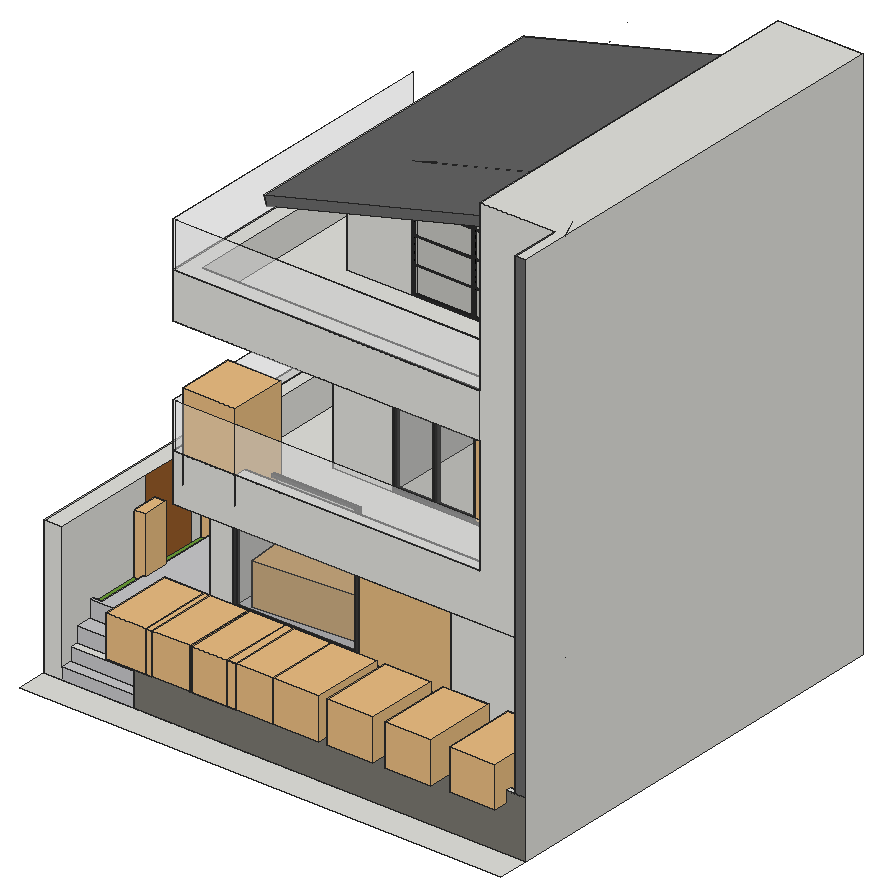
# SketchUp Ruby script. Lengths in inches.
U = 1.inch
M = Sketchup.active_model
def pt(a) = Geom::Point3d.new(a.map { |v| v * U })
def face(e, loops, mat)
  f = e.add_face(loops[0].map { |a| pt(a) })
  loops[1..].each { |l| e.add_face(l.map { |a| pt(a) }).erase! }
  f.material = f.back_material = mat if mat
  f
end
# faces: each face lists its corners as indices into pts; further lists are holes
def faces(e, pts, list, mat = nil) = list.each { |f| face(e, (f[0].is_a?(Array) ? f : [f]).map { |l| l.map { |i| pts[i] } }, mat) }
# xy, xz, yz: faces in a plane at the given z, y or x. An outline is a flat list of corners, or four numbers for a rectangle; further outlines are holes
def ring(l) = l.size == 4 ? [[l[0], l[1]], [l[2], l[1]], [l[2], l[3]], [l[0], l[3]]] : l.each_slice(2).to_a
def flat(e, list, mat, &to3) = list.each { |f| face(e, (f[0].is_a?(Array) ? f : [f]).map { |l| ring(l).map { |u, v| to3.(u, v) } }, mat) }
def xy(e, z, list, mat = nil) = flat(e, list, mat) { |x, y| [x, y, z] }
def xz(e, y, list, mat = nil) = flat(e, list, mat) { |x, z| [x, y, z] }
def yz(e, x, list, mat = nil) = flat(e, list, mat) { |y, z| [x, y, z] }
def lines(e, pts, list) = list.each { |a, b| e.add_line(pt(pts[a]), pt(pts[b])) }
# prism: a flat outline (further loops are holes) pulled along v
def prism(e, loops, v, mat = nil)
  f = face(e, loops, mat); d = Geom::Vector3d.new(v.map { |x| x * U })
  f.pushpull(f.normal.samedirection?(d) ? d.length : -d.length)
end
def box(e, o, s, mat = nil) = prism(e, [[o, [o[0] + s[0], o[1], o[2]], [o[0] + s[0], o[1] + s[1], o[2]], [o[0], o[1] + s[1], o[2]]]], [0, 0, s[2]], mat)
def at(x, y, z, deg = 0) = Geom::Transformation.translation(pt([x, y, z])) * Geom::Transformation.rotation(ORIGIN, Z_AXIS, deg.degrees)
def axes(o, x, y, z) = Geom::Transformation.new([*x, 0, *y, 0, *z, 0, *pt(o).to_a, 1])
def part(name) = M.definitions.add(name)
# library, detail: a bought-in or finely detailed component or shape, given as its bounding box
def library(name, o, s) = part(name).tap { |d| box(d.entities, o, s) }
def detail(e, o, s) = box(e.add_group.entities, o, s)
def put(e, d, t, mat = nil) = e.add_instance(d, t).tap { |i| i.material = mat if mat }
def group(e, t, mat = nil) = e.add_group.tap { |g| g.transformation = t; g.material = mat if mat }.entities
root = M.entities
M.materials.add("Glass_Window_Neutral\#2").color = [0, 0, 0]
M.materials["Glass_Window_Neutral\#2"].alpha = 0.125
M.materials.add("Iron_Blurry_5cm").color = [3, 3, 3]
M.materials.add("Resin FOG").color = [255, 255, 255]
M.materials["Resin FOG"].alpha = 0.29
M.materials.add("[0134_DimGray]").color = [105, 105, 105]
M.materials.add("[Color M07]").color = [58, 58, 58]
M.materials.add("[Color M09]4").color = [0, 0, 0]
M.materials.add("[Grass Dark Green]").color = [106, 157, 55]
M.materials.add("[Polished Concrete New]").color = [200, 200, 203]
M.materials.add("[Rough Square Concrete Block]").color = [123, 120, 113]
M.materials.add("[Slate]").color = [102, 110, 108]
M.materials.add("[Translucent Glass Gray]3").color = [128, 128, 128]
M.materials["[Translucent Glass Gray]3"].alpha = 0.3
M.materials.add("[Wood Floor Dark]").color = [153, 94, 42]
c1 = library("Door+Glass",[-5.91,-81.85,0],[24.58,33.9,83.07])
c2 = part("WINDOW (3)")
xy(c2.entities,0,[[0,0,59.06,1.97]],"[Color M07]")
xy(c2.entities,1.97,[[1.97,0,57.09,0.98],[1.97,0.98,57.09,1.97]],"[Color M07]")
xy(c2.entities,104.33,[[1.97,0,57.09,0.98],[1.97,0.98,57.09,1.97]],"[Color M07]")
xy(c2.entities,106.3,[[0,0,59.06,1.97]],"[Color M07]")
xz(c2.entities,0,[[[0,0,59.06,106.3],[1.97,1.97,57.09,104.33]]],"[Color M07]")
xz(c2.entities,0.98,[[1.97,1.97,57.09,104.33]],"[Translucent Glass Gray]3")
xz(c2.entities,1.97,[[[0,0,59.06,106.3],[1.97,1.97,57.09,104.33]]],"[Color M07]")
yz(c2.entities,0,[[0,0,1.97,106.3]],"[Color M07]")
yz(c2.entities,1.97,[[0,1.97,0.98,104.33],[0.98,1.97,1.97,104.33]],"[Color M07]")
yz(c2.entities,57.09,[[0,1.97,0.98,104.33],[0.98,1.97,1.97,104.33]],"[Color M07]")
yz(c2.entities,59.06,[[0,0,1.97,106.3]],"[Color M07]")
c3 = part("glass")
p = [[-167.89,-148.66,14.5],[-167.89,-148.66,14.51],[-167.89,-148.66,14.52]]
lines(c3.entities,p,[[0,1],[1,2]])
g1 = group(c3.entities,at(-34.63,-28.25,2))
box(g1,[0,0,0],[93.3125,0.375,32.75],"Resin FOG")
c4 = part("Component\#72")
g2 = group(c4.entities,at(0,26.17,94.49),"[Color M09]4")
xy(g2,-94.49,[[0,-26.17,1.18,0]],"Iron_Blurry_5cm")
xy(g2,-93.8,[[0,-25.51,0.59,-0.67],[0.59,-25.51,1.18,-0.67]],"Iron_Blurry_5cm")
xy(g2,-70.52,[[0.59,-25.51,1.18,-0.67]],"Iron_Blurry_5cm")
xy(g2,-69.84,[[0.59,-25.51,1.18,-0.67]],"Iron_Blurry_5cm")
xy(g2,-47.24,[[0.59,-25.51,1.18,-0.67]],"Iron_Blurry_5cm")
xy(g2,-46.56,[[0.59,-25.51,1.18,-0.67]],"Iron_Blurry_5cm")
xy(g2,-23.97,[[0.59,-25.51,1.18,-0.67]],"Iron_Blurry_5cm")
xy(g2,-23.28,[[0.59,-25.51,1.18,-0.67]],"Iron_Blurry_5cm")
xy(g2,-0.6875,[[0,-25.51,0.59,-0.67],[0.59,-25.51,1.18,-0.67]],"Iron_Blurry_5cm")
xy(g2,0,[[0,-26.17,1.18,0]],"Iron_Blurry_5cm")
xz(g2,-26.17,[[0,-94.49,1.18,0]],"Iron_Blurry_5cm")
xz(g2,-25.51,[[0,-93.8,0.59,-0.6875],[0.59,-93.8,1.18,-70.52],[0.59,-70.52,1.18,-69.84],[0.59,-69.84,1.18,-47.24],[0.59,-47.24,1.18,-46.56],
  [0.59,-46.56,1.18,-23.97],[0.59,-23.97,1.18,-23.28],[0.59,-23.28,1.18,-0.6875]],"Iron_Blurry_5cm")
xz(g2,-0.67,[[0,-93.8,0.59,-0.6875],[0.59,-93.8,1.18,-70.52],[0.59,-70.52,1.18,-69.84],[0.59,-69.84,1.18,-47.24],[0.59,-47.24,1.18,-46.56],
  [0.59,-46.56,1.18,-23.97],[0.59,-23.97,1.18,-23.28],[0.59,-23.28,1.18,-0.6875]],"Iron_Blurry_5cm")
xz(g2,0,[[0,-94.49,1.18,0]],"Iron_Blurry_5cm")
yz(g2,0,[[[-26.17,-94.49,0,0],[-25.51,-93.8,-0.67,-0.6875]]],"Iron_Blurry_5cm")
yz(g2,0.59,[[-25.51,-93.8,-0.67,-70.52],[-25.51,-69.84,-0.67,-47.24],[-25.51,-46.56,-0.67,-23.97],[-25.51,-23.28,-0.67,-0.6875]],"Glass_Window_Neutral\#2")
yz(g2,0.59,[[-25.51,-70.52,-0.67,-69.84],[-25.51,-47.24,-0.67,-46.56],[-25.51,-23.97,-0.67,-23.28]],"Iron_Blurry_5cm")
yz(g2,1.18,[[[-26.17,-94.49,0,0],[-25.51,-93.8,-0.67,-0.6875]],[-25.51,-70.52,-0.67,-69.84],[-25.51,-47.24,-0.67,-46.56],[-25.51,-23.97,-0.67,-23.28]],"Iron_Blurry_5cm")
g3 = group(c4.entities,at(0,52.35,94.49),"[Color M09]4")
xy(g3,-94.49,[[0,-26.17,1.18,0]],"Iron_Blurry_5cm")
xy(g3,-93.8,[[0,-25.51,0.59,-0.67],[0.59,-25.51,1.18,-0.67]],"Iron_Blurry_5cm")
xy(g3,-70.52,[[0.59,-25.51,1.18,-0.67]],"Iron_Blurry_5cm")
xy(g3,-69.84,[[0.59,-25.51,1.18,-0.67]],"Iron_Blurry_5cm")
xy(g3,-47.24,[[0.59,-25.51,1.18,-0.67]],"Iron_Blurry_5cm")
xy(g3,-46.56,[[0.59,-25.51,1.18,-0.67]],"Iron_Blurry_5cm")
xy(g3,-23.97,[[0.59,-25.51,1.18,-0.67]],"Iron_Blurry_5cm")
xy(g3,-23.28,[[0.59,-25.51,1.18,-0.67]],"Iron_Blurry_5cm")
xy(g3,-0.6875,[[0,-25.51,0.59,-0.67],[0.59,-25.51,1.18,-0.67]],"Iron_Blurry_5cm")
xy(g3,0,[[0,-26.17,1.18,0]],"Iron_Blurry_5cm")
xz(g3,-26.17,[[0,-94.49,1.18,0]],"Iron_Blurry_5cm")
xz(g3,-25.51,[[0,-93.8,0.59,-0.6875],[0.59,-93.8,1.18,-70.52],[0.59,-70.52,1.18,-69.84],[0.59,-69.84,1.18,-47.24],[0.59,-47.24,1.18,-46.56],
  [0.59,-46.56,1.18,-23.97],[0.59,-23.97,1.18,-23.28],[0.59,-23.28,1.18,-0.6875]],"Iron_Blurry_5cm")
xz(g3,-0.67,[[0,-93.8,0.59,-0.6875],[0.59,-93.8,1.18,-70.52],[0.59,-70.52,1.18,-69.84],[0.59,-69.84,1.18,-47.24],[0.59,-47.24,1.18,-46.56],
  [0.59,-46.56,1.18,-23.97],[0.59,-23.97,1.18,-23.28],[0.59,-23.28,1.18,-0.6875]],"Iron_Blurry_5cm")
xz(g3,0,[[0,-94.49,1.18,0]],"Iron_Blurry_5cm")
yz(g3,0,[[[-26.17,-94.49,0,0],[-25.51,-93.8,-0.67,-0.6875]]],"Iron_Blurry_5cm")
yz(g3,0.59,[[-25.51,-93.8,-0.67,-70.52],[-25.51,-69.84,-0.67,-47.24],[-25.51,-46.56,-0.67,-23.97],[-25.51,-23.28,-0.67,-0.6875]],"Glass_Window_Neutral\#2")
yz(g3,0.59,[[-25.51,-70.52,-0.67,-69.84],[-25.51,-47.24,-0.67,-46.56],[-25.51,-23.97,-0.67,-23.28]],"Iron_Blurry_5cm")
yz(g3,1.18,[[[-26.17,-94.49,0,0],[-25.51,-93.8,-0.67,-0.6875]],[-25.51,-70.52,-0.67,-69.84],[-25.51,-47.24,-0.67,-46.56],[-25.51,-23.97,-0.67,-23.28]],"Iron_Blurry_5cm")
c5 = library("SOFA\#1",[0.35,-39.08,0.31],[80.46,34.29,30.24])
c6 = library("CURTAIN",[20.4,9.88,0],[29.77,2.88,102.36])
c7 = library("S21",[-74.41,-56.05,0],[89.11,79.55,33.18])
c8 = library("Broadleaf plant",[0,0,0],[149.19,166.1,98.1875])
c9 = library("cay+chuoi",[26.89,19.66,0.52],[41.96,45.65,69.71])
c10 = library("Group_2",[-1.28,-0.39,0],[21.22,20.51,48.44])
xy(root,0,[[0,0,384.5625,24.3],[0,24.3,370.25,361.1875],[370.25,24.3,384.5625,49.12],[370.25,49.12,384.5625,361.1875]])
xy(root,9.26,[[13.89,24.3,71.28,33.18]],"[Polished Concrete New]")
xy(root,15.375,[[75.74,28.76,380.11,44.66]])
xy(root,19.65,[[13.89,33.18,71.28,39.8]])
xy(root,31.63,[[13.89,39.8,71.28,52.87]],"[Polished Concrete New]")
xy(root,41.75,[[13.89,54.78,21.5625,334.58]],"[Grass Dark Green]")
xy(root,45.625,[[71.28,24.3,376.39,24.3,376.39,28.76,75.74,28.76,75.74,44.66,376.39,44.66,376.39,49.12,71.28,49.12],[376.39,24.3,380.11,28.76]])
xy(root,45.625,[[71.28,49.12,376.39,49.12,376.39,81.5,278.92,81.5,278.92,167.87,89.95,167.87,89.95,100.12,71.28,100.12,71.28,334.58,21.5625,334.58,21.5625,54.78,13.89,54.78,13.89,52.87,71.28,52.87]],"[Polished Concrete New]")
xy(root,45.625,[[376.39,28.76,380.11,44.66]],"[Slate]")
xy(root,109.1875,[[0,24.3,13.89,361.1875],[13.89,334.58,71.28,361.1875]])
xy(root,128.75,[[71.28,63.93,89.95,100.12],[89.95,63.93,168.05,167.87],[168.05,63.93,168.05,167.87,278.92,167.87,278.92,81.5,238.99,81.5,238.99,63.93],[238.99,63.93,318.92,81.5],[318.92,63.93,376.39,81.5]])
xy(root,138.125,[[81.53,73.41,316.72,73.41,316.72,148.24,277.01,148.24,277.01,335.05,179.52,335.05,179.52,148.24,131.1,148.24,131.1,340.9,81.53,340.9]])
xy(root,166.625,[[71.28,63.93,316.72,63.93,316.72,73.41,81.53,73.41,81.53,361.1875,71.28,361.1875]])
xy(root,259.91,[[179.52,148.24,277.01,335.05]])
xy(root,259.91,[[71.28,63.93,71.28,361.1875,81.53,361.1875,81.53,340.9,131.1,340.9,131.1,63.93],[131.1,63.93,316.72,148.24]],"[Wood Floor Dark]")
xy(root,270.4375,[[83.91,77.46,316.72,77.46,316.72,167.52,277.01,167.52,277.01,171.89,179.52,171.89,179.52,167.52,127.35,167.52,127.35,349.08,316.72,361.1875,83.91,361.1875],[127.35,349.08,316.72,349.08,316.72,361.1875]])
xy(root,295.9375,[[71.28,63.93,316.72,63.93,316.72,77.46,83.91,77.46,83.91,361.1875,71.28,361.1875]])
xy(root,430.4375,[[376.39,24.3,384.5625,24.3,384.5625,361.1875,316.72,361.1875,316.72,63.93,376.39,63.93]])
xz(root,24.3,[[0,0,13.89,109.1875]])
xz(root,24.3,[[376.39,45.625,384.5625,430.4375]],"[0134_DimGray]")
xz(root,24.3,[[13.89,0,71.28,9.26]],"[Polished Concrete New]")
xz(root,24.3,[[71.28,0,384.5625,45.625]],"[Rough Square Concrete Block]")
xz(root,28.76,[[75.74,15.375,380.11,45.625]])
xz(root,33.18,[[13.89,9.26,71.28,19.65]],"[Polished Concrete New]")
xz(root,39.8,[[13.89,19.65,71.28,31.63]],"[Polished Concrete New]")
xz(root,44.66,[[75.74,15.375,380.11,45.625]])
xz(root,52.87,[[13.89,31.63,71.28,45.625]],"[Polished Concrete New]")
xz(root,54.78,[[13.89,41.75,21.5625,45.625]],"[Polished Concrete New]")
xz(root,63.93,[[71.28,128.75,376.39,128.75,376.39,430.4375,316.72,430.4375,316.72,166.625,71.28,166.625],[71.28,259.91,316.72,295.9375]])
xz(root,73.41,[[81.53,138.125,316.72,166.625]])
xz(root,77.46,[[83.91,270.4375,316.72,295.9375]])
xz(root,81.5,[[278.92,45.625,376.39,128.75]])
xz(root,99.1,[[117.72,342.48,317.8,396.09,315.85,403.37,115.77,349.76]],"[0134_DimGray]")
xz(root,100.12,[[71.28,45.625,89.95,128.75]])
xz(root,148.24,[[131.1,138.125,179.52,259.91],[277.01,138.125,316.72,259.91]])
xz(root,167.52,[[127.35,270.4375,179.52,270.4375,179.52,359.04,277.01,385.16,277.01,270.4375,316.72,270.4375,316.72,395.1875,285.33,395.1875,239.34,382.88,191.55,370.0625,187.79,369.05,176.96,364.52,176.85,364.83,127.23,346.03,127.35,345.72],[187.79,369.05,191.55,370.0625,191.55,370.09,187.96,369.125],[191.55,370.0625,239.34,382.88,191.55,370.09],[191.55,370.0625,239.34,382.88,191.55,370.09]])
xz(root,167.87,[[89.95,45.625,164.47,128.75]])
xz(root,167.87,[[164.47,45.625,278.92,128.75]],"[Wood Floor Dark]")
xz(root,171.89,[[179.52,270.4375,277.01,270.4375,277.01,385.16,179.52,359.04]])
xz(root,334.58,[[13.89,41.75,21.5625,41.75,21.5625,45.625,71.28,45.625,71.28,109.1875,13.89,109.1875]])
xz(root,335.05,[[179.52,138.125,277.01,259.91]])
xz(root,340.9,[[81.53,138.125,131.1,259.91]])
xz(root,349.08,[[127.35,345.72,127.23,346.03,127.35,346.07],[127.35,345.72,127.35,346.07,176.85,364.83]])
xz(root,358.27,[[117.72,342.48,115.77,349.76,315.85,403.37,317.8,396.09]])
xz(root,361.1875,[[0,0,0,109.1875,71.28,109.1875,71.28,166.625,81.53,166.625,81.53,259.91,71.28,259.91,71.28,295.9375,83.91,295.9375,83.91,270.4375,142.5625,270.4375,142.5625,0],[142.5625,0,142.5625,270.4375,316.72,270.4375,316.72,430.4375,384.5625,430.4375,384.5625,0]])
yz(root,0,[[24.3,0,361.1875,109.1875]])
yz(root,13.89,[[24.3,9.26,33.18,9.26,33.18,19.65,39.8,19.65,39.8,31.63,52.87,31.63,52.87,45.625,54.78,45.625,54.78,41.75,107.85,41.75,107.85,109.1875,24.3,109.1875],[154.01,41.75,198.21,109.1875],[258.15,41.75,334.58,109.1875]])
yz(root,13.89,[[107.85,41.75,154.01,109.1875],[198.21,41.75,258.15,109.1875]],"[Wood Floor Dark]")
yz(root,21.5625,[[54.78,41.75,334.58,45.625]],"[Polished Concrete New]")
yz(root,71.28,[[24.3,0,24.3,9.26,33.18,9.26,33.18,12.26,49.12,12.26,49.12,0],[24.3,9.26,33.18,12.26],[24.3,12.26,33.18,21.58],[33.18,19.65,33.18,21.58,24.3,21.58,24.3,45.625,49.12,45.625,49.12,31.63,39.8,31.63,39.8,19.65],[39.8,24.52,49.12,31.63],
  [49.12,31.63,52.87,45.625],[100.12,45.625,100.12,128.75,63.93,128.75,63.93,166.625,361.1875,166.625,361.1875,109.1875,334.58,109.1875,334.58,45.625],[63.93,259.91,361.1875,295.9375]])
yz(root,75.74,[[28.76,15.375,44.66,45.625]])
yz(root,81.53,[[73.41,138.125,340.9,166.625],[340.9,166.625,361.1875,259.91]])
yz(root,83.91,[[77.46,270.4375,361.1875,295.9375]])
yz(root,89.95,[[100.12,45.625,167.87,128.75]])
yz(root,127.35,[[167.52,270.4375,349.08,345.72]])
yz(root,131.1,[[148.24,138.125,340.9,259.91]])
yz(root,179.52,[[148.24,138.125,335.05,259.91],[167.52,270.4375,171.89,358.25],[167.52,358.25,171.89,358.87],[167.52,358.87,171.89,359.04]])
yz(root,277.01,[[148.24,138.125,335.05,259.91],[167.52,270.4375,171.89,385.16]])
yz(root,278.92,[[81.5,45.625,167.87,128.75]])
yz(root,316.72,[[73.41,138.125,73.41,166.625,63.93,166.625,63.93,259.91,148.24,259.91,148.24,138.125],[77.46,270.4375,77.46,295.9375,63.93,295.9375,63.93,430.4375,361.1875,430.4375,361.1875,270.4375,349.08,270.4375,349.08,395.1875,167.52,395.1875,167.52,270.4375]])
yz(root,376.39,[[24.3,45.625,24.3,430.4375,63.93,430.4375,63.93,128.75,81.5,128.75,81.5,45.625]],"[0134_DimGray]")
yz(root,380.11,[[28.76,15.375,44.66,45.625]])
yz(root,384.5625,[[24.3,0,361.1875,430.4375]])
p = [[127.35,349.08,270.4375],[127.35,349.08,345.72],[127.35,349.08,346.07],[127.35,349.08,349.9],[316.72,361.1875,349.9],[316.72,361.1875,270.4375],
  [117.72,358.27,342.48],[117.72,99.1,342.48],[115.77,99.1,349.76],[115.77,358.27,349.76],[317.8,358.27,396.09],[317.8,99.1,396.09],
  [179.52,167.52,359.04],[277.01,167.52,385.16],[277.01,171.89,385.16],[179.52,171.89,359.04],[127.35,167.52,345.72],[127.23,167.52,346.03],
  [127.23,349.08,346.03],[176.85,167.52,364.83],[176.85,349.08,364.83],[315.85,99.1,403.37],[315.85,358.27,403.37],[176.96,167.52,364.52],
  [176.96,349.08,364.52],[316.72,349.08,395.1875],[285.33,349.08,395.1875],[191.55,167.52,369.1875],[191.55,167.52,370.0625],[191.55,349.95,376.35],
  [191.55,349.08,376.35],[178.89,167.52,358.87],[179.52,167.52,366.84],[187.79,167.52,369.05],[384.5625,63.93,430.4375],[376.39,81.5,430.4375],
  [376.39,81.5,128.75],[384.5625,63.93,128.75]]
faces(root,p,[[0,1,2,3,4,5],[6,7,8,9],[1,16,17,18],[18,17,19,20,2],[13,12,15,14],[23,24,20,19],[11,10,22,21]])
faces(root,p,[[[7,6,10,11],[12,13,14,15]]],"[Wood Floor Dark]")
faces(root,p,[[9,8,21,22]],"[0134_DimGray]")
lines(root,p,[[25,26],[27,28],[29,30],[12,31],[32,33],[34,35],[35,36],[36,37]])
put(root,c1,axes([53.29,120.77,45.625],[0.10626,0.99434,0],[-2.88358,0.30817,0],[0,0,1]))
put(root,c2,axes([89.95,100.12,45.625],[1.71,0,0],[0,1,0],[0,0,1]))
put(root,c3,axes([163.55,88.23,293.71],[2.60999,0,0],[0,0.86,0],[0,0,1.115]))
put(root,c3,axes([163.55,88.23,164.4],[2.60999,0,0],[0,0.86,0],[0,0,1.115]))
put(root,c3,axes([95.58,215.03,293.71],[0,-2.57471,0],[0.86,0,0],[0,0,1.115]))
put(root,c3,axes([95.58,215.03,164.4],[0,-2.57471,0],[0.86,0,0],[0,0,1.115]))
put(root,c4,axes([277.01,167.52,270.4375],[0,1,0],[-1.8623,0,0],[0,0,0.9044]))
put(root,c5,at(190.06,295.82,142.24))
put(root,c6,axes([222.82,104.33,140.38],[1.05822,0,0],[0,4.44245,0],[0,0,1.16768]))
put(root,c6,axes([227.52,145.53,261.63],[1,0,0],[0,2.22481,0],[0,0,0.92086]))
put(root,c7,axes([119.9375,145.91,45.625],[-0.03923,0.49846,0],[-0.99692,-0.07846,0],[0,0,1]))
put(root,c8,axes([65.69,4.17,42.14],[0.245,0,0],[0,0.35,0],[0,0,0.3332]))
put(root,c8,axes([97.5,4.17,42.14],[0.245,0,0],[0,0.35,0],[0,0,0.3332]))
put(root,c8,axes([132.81,4.17,42.14],[0.245,0,0],[0,0.35,0],[0,0,0.3332]))
put(root,c8,axes([162.31,4.17,42.14],[0.245,0,0],[0,0.35,0],[0,0,0.3332]))
put(root,c8,axes([198.94,4.17,42.14],[0.245,0,0],[0,0.35,0],[0,0,0.3332]))
put(root,c8,axes([242.06,4.17,42.14],[0.245,0,0],[0,0.35,0],[0,0,0.3332]))
put(root,c8,axes([288.37,4.17,42.14],[0.245,0,0],[0,0.35,0],[0,0,0.3332]))
put(root,c8,axes([331.94,14.16,35.45],[0.245,0,0],[0,0.35,0],[0,0,0.3332]))
put(root,c9,at(51.74,44.27,143.99))
put(root,c10,axes([14.71,96.87,41.75],[0.42201,0,0],[0,1,0],[0,0,1]))
put(root,c10,axes([14.71,163.05,41.75],[0.42201,0,0],[0,1,0],[0,0,1]))
put(root,c10,axes([14.71,273.87,41.75],[0.42201,0,0],[0,1,0],[0,0,1]))
g4 = group(root,at(179.52,148.24,-20.12))
put(g4,c2,axes([64.65,0,158.24],[0.5561,0,0],[0,2.29,0],[0,0,1.14565]))
put(g4,c2,axes([32.5,0,158.24],[0.5561,0,0],[0,2.29,0],[0,0,1.14565]))
put(g4,c2,axes([0,0,158.24],[0.5561,0,0],[0,2.29,0],[0,0,1.14565]))
